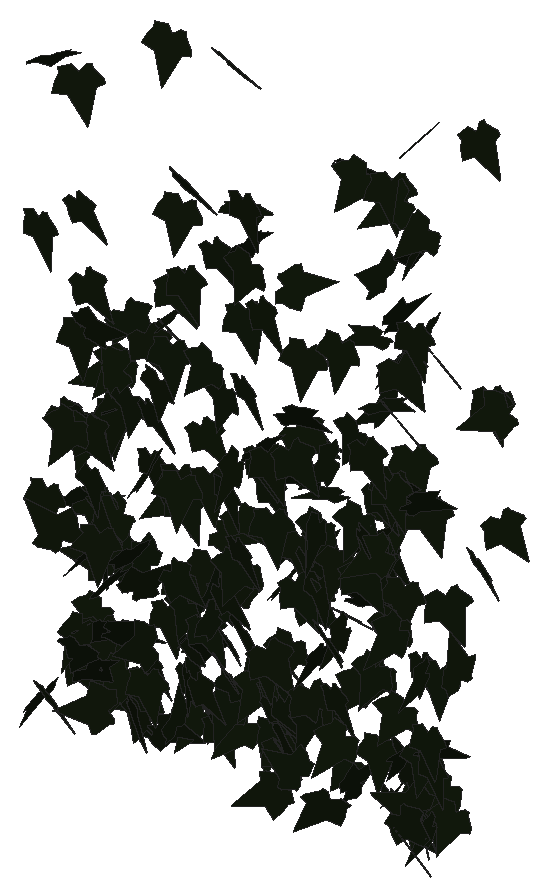
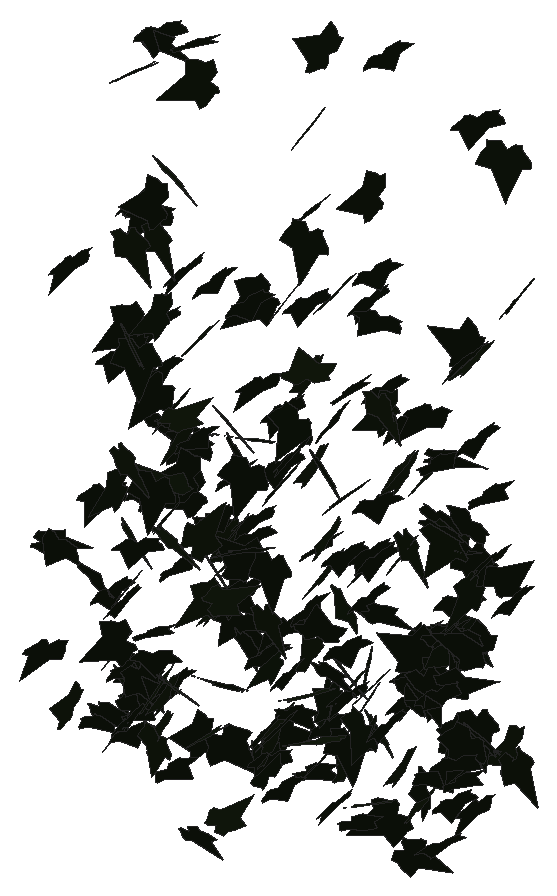
# SketchUp Ruby script. Lengths in inches.
U = 1.inch
M = Sketchup.active_model
def pt(a) = Geom::Point3d.new(a.map { |v| v * U })
def face(e, loops, mat)
  f = e.add_face(loops[0].map { |a| pt(a) })
  loops[1..].each { |l| e.add_face(l.map { |a| pt(a) }).erase! }
  f.material = f.back_material = mat if mat
  f
end
# faces: each face lists its corners as indices into pts; further lists are holes
def faces(e, pts, list, mat = nil) = list.each { |f| face(e, (f[0].is_a?(Array) ? f : [f]).map { |l| l.map { |i| pts[i] } }, mat) }
# xy, xz, yz: faces in a plane at the given z, y or x. An outline is a flat list of corners, or four numbers for a rectangle; further outlines are holes
def ring(l) = l.size == 4 ? [[l[0], l[1]], [l[2], l[1]], [l[2], l[3]], [l[0], l[3]]] : l.each_slice(2).to_a
def flat(e, list, mat, &to3) = list.each { |f| face(e, (f[0].is_a?(Array) ? f : [f]).map { |l| ring(l).map { |u, v| to3.(u, v) } }, mat) }
def xy(e, z, list, mat = nil) = flat(e, list, mat) { |x, y| [x, y, z] }
def xz(e, y, list, mat = nil) = flat(e, list, mat) { |x, z| [x, y, z] }
def yz(e, x, list, mat = nil) = flat(e, list, mat) { |y, z| [x, y, z] }
def lines(e, pts, list) = list.each { |a, b| e.add_line(pt(pts[a]), pt(pts[b])) }
# prism: a flat outline (further loops are holes) pulled along v
def prism(e, loops, v, mat = nil)
  f = face(e, loops, mat); d = Geom::Vector3d.new(v.map { |x| x * U })
  f.pushpull(f.normal.samedirection?(d) ? d.length : -d.length)
end
def box(e, o, s, mat = nil) = prism(e, [[o, [o[0] + s[0], o[1], o[2]], [o[0] + s[0], o[1] + s[1], o[2]], [o[0], o[1] + s[1], o[2]]]], [0, 0, s[2]], mat)
def at(x, y, z, deg = 0) = Geom::Transformation.translation(pt([x, y, z])) * Geom::Transformation.rotation(ORIGIN, Z_AXIS, deg.degrees)
def axes(o, x, y, z) = Geom::Transformation.new([*x, 0, *y, 0, *z, 0, *pt(o).to_a, 1])
def part(name) = M.definitions.add(name)
# library, detail: a bought-in or finely detailed component or shape, given as its bounding box
def library(name, o, s) = part(name).tap { |d| box(d.entities, o, s) }
def detail(e, o, s) = box(e.add_group.entities, o, s)
def put(e, d, t, mat = nil) = e.add_instance(d, t).tap { |i| i.material = mat if mat }
def group(e, t, mat = nil) = e.add_group.tap { |g| g.transformation = t; g.material = mat if mat }.entities
root = M.entities
M.materials.add("efeu1").color = [18, 25, 13]
c1 = part("ivyleaf_9")
p = [[1.54,2.16,1.25],[1.36,2.04,1.19],[-0.21,0.99,0.68],[-0.71,1.11,0.82],[-0.85,0.86,0.67],[-0.8,0.17,0.21],
  [-0.9,-0.01,0.1],[-0.67,-0.16,-0.02],[-0.08,-0.08,-0.05],[-0.03,-0.6,-0.4],[0.65,-0.88,-0.66],[0.83,-0.6,-0.49],
  [1.29,-0.42,-0.43],[1.8125,-0.07,-0.26],[1.21,0.44,0.15]]
faces(c1.entities,p,[[0,1,2,3,4,5,6,7,8,9,10,11,12,13,14]],"efeu1")
put(root,c1,axes([586.22,116.61,357.54],[0.71819,-0.99518,-0.77753],[-0.16369,0.81357,-1.1925],[1.25226,0.6771,0.29005]))
put(root,c1,axes([586.3,123.58,334],[-0.07345,-1.46368,-0.26729],[0.34823,0.24327,-1.42785],[1.44656,-0.13288,0.33015]))
put(root,c1,axes([586.64,118.75,355.34],[1.33189,-0.02046,-0.50214],[-0.4908,0.25288,-1.31212],[0.10806,1.40076,0.22954]))
put(root,c1,axes([587.66,113.28,392.88],[0.45263,1.4208,-0.19565],[-0.46923,-0.04716,-1.42808],[-1.35527,0.49085,0.4291]))
put(root,c1,axes([586.53,118.27,376.59],[0.90416,-1.0969,-0.2869],[0.04377,0.40045,-1.3931],[1.13296,0.85992,0.28278]))
put(root,c1,axes([587.42,120.06,337.79],[-0.70992,-1.06443,0.44559],[-0.10133,-0.46364,-1.26898],[1.14948,-0.69826,0.16333]))
put(root,c1,axes([587.125,113.47,351.75],[0.0436,-1.41863,0.05695],[0.00445,-0.05684,-1.4193],[1.41977,0.04374,0.0027]))
put(root,c1,axes([588.15,117.21,357.48],[0.83336,0.45387,-1.07421],[-0.90735,-0.57701,-0.94772],[-0.73255,1.23104,-0.04816]))
put(root,c1,axes([587.53,117.22,334.38],[0.41458,-0.9867,-0.84246],[-0.20487,0.82354,-1.06536],[1.28115,0.45099,0.10225]))
put(root,c1,axes([587.21,117.31,348.66],[0.5196,-0.16158,1.32532],[1.32539,0.23386,-0.49112],[-0.16095,1.40419,0.2343]))
put(root,c1,axes([589.23,110.3125,334.82],[-0.63267,1.1754,-0.62675],[0.22482,-0.58968,-1.33281],[-1.31295,-0.66735,0.07379]))
put(root,c1,axes([588.08,111.31,378.49],[0.49863,-1.42704,0.04607],[-0.00245,-0.04966,-1.51153],[1.42778,0.49828,-0.01868]))
put(root,c1,axes([588.76,117.14,356.88],[-1.03775,-0.88039,-0.44682],[0.38444,0.23674,-1.35934],[0.90936,-1.10477,0.06478]))
put(root,c1,axes([590.22,117.6,344.51],[-0.65379,0.04671,1.2732],[-1.26249,-0.21614,-0.64036],[0.17128,-1.41484,0.13986]))
put(root,c1,axes([588.86,117.71,349.93],[-0.82625,-0.6682,-0.95212],[0.72316,0.61967,-1.06243],[0.91108,-1.09783,-0.02017]))
put(root,c1,axes([588.67,117.31,352.26],[0.41477,-1.29731,0.38748],[0.11544,-0.36989,-1.362],[1.34901,0.43052,-0.00258]))
put(root,c1,axes([589.17,118.33,334.66],[-0.23341,-1.27695,-0.30092],[0.05641,0.2956,-1.2981],[1.31071,-0.24012,0.00228]))
put(root,c1,axes([589.55,114.96,339.24],[-1.19802,-0.32954,-0.68957],[0.73792,-0.16502,-1.20316],[0.19894,-1.37241,0.31025]))
put(root,c1,axes([589.22,115.3125,366.79],[0.03639,-1.47553,-0.11222],[-0.03578,0.11134,-1.47561],[1.47935,0.03899,-0.03293]))
put(root,c1,axes([589.38,117.78,337.9],[-0.33749,-1.1931,-0.69454],[0.22667,0.6574,-1.23944],[1.3618,-0.4051,0.03418]))
put(root,c1,axes([589.84,115.43,338.71],[0.78837,1.16892,0.14934],[0.07963,0.12643,-1.40993],[-1.17573,0.79237,0.00465]))
put(root,c1,axes([589.78,119.55,344.96],[-0.10207,-1.26752,-0.5716],[0.04327,0.56997,-1.27162],[1.38977,-0.11084,-0.00239]))
put(root,c1,axes([590.11,117.13,358.24],[1.00117,1.09817,0.29768],[-0.05991,0.44685,-1.44695],[-1.13622,0.94408,0.3386]))
put(root,c1,axes([590.17,118.1,349.35],[-0.40572,-1.16314,0.63076],[-0.07215,-0.63932,-1.22533],[1.32119,-0.3921,0.12678]))
put(root,c1,axes([591.28,110.08,350.23],[0.18792,0.30059,1.46884],[-1.48233,0.25923,0.1366],[-0.22482,-1.45795,0.32713]))
put(root,c1,axes([591.62,121.27,330.4375],[-0.2193,-0.15658,-1.36819],[-0.82869,-1.09151,0.25774],[-1.09988,0.8536,0.07861]))
put(root,c1,axes([591.31,117.95,349],[-1.16937,-0.64385,0.53498],[-0.46293,-0.26836,-1.33486],[0.69745,-1.25762,0.01095]))
put(root,c1,axes([590.69,112.47,359.73],[-0.61427,-1.2618,0.47841],[-0.10896,-0.47755,-1.39944],[1.34505,-0.61494,0.10512]))
put(root,c1,axes([589.83,109.71,335.49],[1.16984,-0.88217,0.28166],[0.23188,-0.16031,-1.46513],[0.89655,1.19254,0.01141]))
put(root,c1,axes([591.32,112.62,338.86],[0.76274,0.60119,-1.10895],[-0.96426,-0.55762,-0.96552],[-0.81326,1.22499,0.10473]))
put(root,c1,axes([590.06,127.95,338.22],[-0.05013,-1.39465,-0.24492],[0.77061,0.17873,-1.17548],[1.18794,-0.1748,0.7522]))
put(root,c1,axes([591.68,118.86,345.28],[-0.16332,1.30316,-0.58109],[-0.03806,-0.58866,-1.30942],[-1.42634,-0.13351,0.10148]))
put(root,c1,axes([591.88,113.99,347.84],[-0.72942,1.02361,-0.70913],[0.04516,-0.79955,-1.20058],[-1.24443,-0.629,0.37209]))
put(root,c1,axes([590.64,116.51,344.31],[-0.09897,0.18185,1.45176],[0.32329,-1.4164,0.19946],[1.42694,0.33352,0.05551]))
put(root,c1,axes([590.97,117.73,358.95],[-0.86623,-0.79984,-0.90298],[0.92176,0.2782,-1.13067],[0.77812,-1.21997,0.33418]))
put(root,c1,axes([590.46,114.52,358.34],[-0.13441,-0.56577,-1.35578],[1.18838,0.75854,-0.43436],[0.8637,-1.13174,0.38665]))
put(root,c1,axes([592.55,120,343.84],[-0.46042,0.32471,1.30651],[-1.07342,0.74482,-0.56339],[-0.81251,-1.16799,0.00394]))
put(root,c1,axes([591.2,113.52,373],[0.66268,-1.15667,-0.60639],[-0.03577,0.66366,-1.305],[1.30549,0.60532,0.27205]))
put(root,c1,axes([591.79,117.18,359.67],[-1.16008,-0.43014,-0.81683],[0.77741,0.25228,-1.23694],[0.49786,-1.39619,0.02814]))
put(root,c1,axes([592.93,115.95,363.93],[-1.22716,-0.12721,0.85092],[-0.80276,-0.36399,-1.21213],[0.30955,-1.44827,0.2299]))
put(root,c1,axes([592.32,117.07,364.11],[-0.79306,-1.07983,0.55135],[-0.20758,-0.52817,-1.33301],[1.19455,-0.80868,0.1344]))
put(root,c1,axes([592.28,112.46,337.17],[0.79684,1.17437,0.25341],[0.11681,0.2269,-1.41887],[-1.1957,0.80479,0.03026]))
put(root,c1,axes([592.15,111.47,393.59],[-0.31415,-1.32015,-0.67244],[0.17383,0.6498,-1.35691],[1.47131,-0.35864,0.01674]))
put(root,c1,axes([592.7,116.78,335.25],[-0.86334,-1.22428,0.02958],[-0.01057,-0.02874,-1.49805],[1.22459,-0.86337,0.00792]))
put(root,c1,axes([592.96,113.13,349.7],[-0.45901,-1.28293,-0.40304],[0.1232,0.38397,-1.36251],[1.33909,-0.47508,-0.0128]))
put(root,c1,axes([592.61,116.99,368.77],[0.22659,-0.81784,-1.18014],[0.18579,1.2014,-0.7969],[1.42375,-0.02662,0.29181]))
put(root,c1,axes([593.49,112.73,345.13],[0.54595,0.90484,1.05669],[0.21228,1.06766,-1.02392],[-1.37486,0.52415,0.26151]))
put(root,c1,axes([594.45,112.05,334.28],[-0.83948,-0.18439,1.19989],[-1.13496,-0.39852,-0.85529],[0.43083,-1.40913,0.08488]))
put(root,c1,axes([593.3,128.61,343.36],[1.22881,-0.55122,-0.41885],[0.3017,1.1944,-0.68674],[0.6231,0.50872,1.15853]))
put(root,c1,axes([593.81,117.28,331.58],[-0.05729,-1.07996,0.85608],[0.25628,-0.85023,-1.05542],[1.35407,0.11523,0.23597]))
put(root,c1,axes([593.93,116.16,361.6],[0.02406,-1.2772,0.64928],[0.19948,-0.64006,-1.26646],[1.41881,0.11165,0.16705]))
put(root,c1,axes([595.4,120.93,351.04],[-1.22157,-0.39612,0.48577],[-0.46186,-0.15052,-1.28419],[0.42375,-1.30597,0.00067]))
put(root,c1,axes([594.05,118.37,336.25],[0.87876,-1.00952,-0.04734],[-0.02769,0.03866,-1.33841],[1.01025,0.87919,0.00449]))
put(root,c1,axes([595.72,116.36,355.59],[-0.95245,1.0759,-0.2968],[0.20577,-0.21422,-1.43686],[-1.09695,-0.97436,-0.01183]))
put(root,c1,axes([594.18,115.65,332.76],[-0.01391,0.03691,-1.4553],[1.45574,0.0082,-0.01371],[0.00785,-1.45534,-0.03698]))
put(root,c1,axes([594.02,110.16,370.88],[0.51863,-0.22234,1.37144],[1.23485,-0.59711,-0.56379],[0.63673,1.33913,-0.02368]))
put(root,c1,axes([594.59,117.94,355.4],[0.57722,-1.29926,0.06332],[0.02392,-0.05866,-1.42171],[1.30059,0.57772,-0.00195]))
put(root,c1,axes([594.84,119.82,340.4],[0.22889,-1.3565,-0.16098],[-0.0017,0.16294,-1.37544],[1.36601,0.22749,0.02526]))
put(root,c1,axes([594.8125,117.05,367.39],[0.29106,-1.201,-0.72711],[0.18321,0.76872,-1.19638],[1.39196,0.14995,0.30951]))
put(root,c1,axes([596.44,118.73,369.22],[-0.60027,1.30334,0.11699],[-0.30422,-0.01381,-1.40712],[-1.27273,-0.61141,0.28116]))
put(root,c1,axes([595.07,118.26,362.64],[0.16605,-1.25244,0.68003],[0.20928,-0.65578,-1.25887],[1.40969,0.24489,0.10679]))
put(root,c1,axes([595.11,115.16,344.48],[0.11476,-0.21163,1.43679],[1.36908,0.49664,-0.0362],[-0.48455,1.3531,0.238]))
put(root,c1,axes([595.24,112.08,341.9],[1.18145,0.239,0.91451],[0.87298,0.28542,-1.20239],[-0.36244,1.46653,0.08497]))
put(root,c1,axes([595.67,117.72,330.75],[0.06905,0.21885,-1.43136],[0.55156,1.32098,0.22858],[1.33883,-0.55549,-0.02035]))
put(root,c1,axes([596.18,120.57,351.99],[0.06787,-1.36175,-0.14946],[-0.0087,0.14921,-1.36344],[1.3699,0.06842,-0.00126]))
put(root,c1,axes([595.98,115.74,361.63],[1.05883,-1.02786,-0.12884],[-0.05951,0.12358,-1.47492],[1.03419,1.05946,0.04704]))
put(root,c1,axes([595.92,118.14,368.18],[1.27409,-0.60733,0.25545],[0.26186,-0.04354,-1.40959],[0.60459,1.29872,0.0722]))
put(root,c1,axes([597.3125,119.67,339.2],[0.13338,1.21568,0.7693],[-0.04756,0.7759,-1.21787],[-1.43786,0.0871,0.11164]))
put(root,c1,axes([595.94,127.86,346.26],[0.6012,-1.23103,-0.37042],[0.63406,0.63968,-1.09676],[1.11831,0.29912,0.82098]))
put(root,c1,axes([597.37,120.99,331.01],[-0.90845,-0.9713,0.2073],[-0.0564,-0.23003,-1.32498],[0.99157,-0.90296,0.11455]))
put(root,c1,axes([596.89,118.61,354.49],[0.10619,-1.39244,-0.29469],[-0.03417,0.29293,-1.39643],[1.42287,0.11095,-0.01154]))
put(root,c1,axes([596.58,127.91,375.36],[-0.29007,-1.43899,0.38433],[1.17655,-0.46147,-0.83983],[0.9133,0.13746,1.20396]))
put(root,c1,axes([598.15,120.41,338.24],[0.37869,1.19675,-0.49344],[-0.21519,-0.44877,-1.25355],[-1.27647,0.43069,0.06494]))
put(root,c1,axes([597.46,119.0625,342.15],[-0.16987,-1.19487,0.69858],[0.13361,-0.71469,-1.18994],[1.37763,-0.07802,0.20155]))
put(root,c1,axes([597.24,119.77,337.9],[0.43448,-1.13903,0.66149],[0.22676,-0.62146,-1.21905],[1.29751,0.49002,-0.00845]))
put(root,c1,axes([597.82,117.86,380.34],[-0.4341,-1.39095,-0.09361],[0.02466,0.09036,-1.45711],[1.39387,-0.43479,-0.00337]))
put(root,c1,axes([598.38,112.65,338.41],[0.08376,-1.39141,-0.30198],[0.01948,0.30359,-1.39344],[1.42367,0.0777,0.03683]))
put(root,c1,axes([598.63,115.55,368.27],[-0.09613,-1.44563,-0.17645],[0.02497,0.17517,-1.44876],[1.45615,-0.09844,0.0132]))
put(root,c1,axes([598.98,120.16,346.22],[-0.43427,-1.31166,-0.15494],[0.03289,0.15231,-1.38159],[1.32037,-0.4352,-0.01654]))
put(root,c1,axes([599.49,111.63,342.22],[-0.45485,-0.48635,1.32151],[-0.64146,-1.16472,-0.64944],[1.25358,-0.77246,0.14718]))
put(root,c1,axes([598.8,116.91,353.75],[0.20587,-1.34072,-0.43835],[0.0723,0.45244,-1.34986],[1.40871,0.17271,0.13334]))
put(root,c1,axes([599.42,114.5,398.35],[-0.37937,-1.46477,0.04473],[-0.00666,-0.04448,-1.51309],[1.46544,-0.3794,0.0047]))
put(root,c1,axes([599.3,119.66,354.57],[-0.11988,-1.35425,-0.37068],[0.09334,0.36352,-1.35827],[1.40095,-0.1401,0.05878]))
put(root,c1,axes([599,115.55,374.62],[-0.24017,-0.98003,-1.02974],[0.80127,0.7693,-0.91904],[1.17421,-0.72541,0.41653]))
put(root,c1,axes([599.38,118.9,341.28],[0.33076,-1.22251,-0.58126],[0.04295,0.60754,-1.25334],[1.35298,0.27958,0.18189]))
put(root,c1,axes([599.45,118.58,359.67],[0.65155,-1.18582,-0.46502],[0.13358,0.58306,-1.29966],[1.26671,0.54846,0.37624]))
put(root,c1,axes([601.12,113.13,334.8],[-1.11212,0.5975,-0.80749],[-0.73591,0.33534,1.26168],[0.68372,1.33281,0.04455]))
put(root,c1,axes([599.89,120.03,331.43],[0.4062,-1.22151,-0.33495],[0.01537,0.35648,-1.28139],[1.2665,0.38745,0.12298]))
put(root,c1,axes([601.19,120.0625,343.4375],[-1.35913,-0.13324,-0.0068],[0.0076,-0.00781,-1.36562],[0.13319,-1.35913,0.00851]))
put(root,c1,axes([600.36,114.53,356.7],[-0.45459,-1.33089,-0.26563],[0.12181,0.23899,-1.40589],[1.35166,-0.46914,0.03736]))
put(root,c1,axes([599.8,118.5,334.08],[0.36086,-0.99137,0.89218],[0.51927,-0.7469,-1.03996],[1.22848,0.60692,0.17751]))
put(root,c1,axes([601.45,117.88,342.93],[-1.19388,0.63723,0.09578],[-0.09041,0.03402,-1.35324],[-0.63801,-1.19723,0.01253]))
put(root,c1,axes([600.3,115.4,338.71],[0.87639,-1.01627,-0.57294],[-0.36824,0.439,-1.34194],[1.10701,0.95058,0.0072]))
put(root,c1,axes([600.3,115.1875,375.79],[0.26162,-1.37055,-0.38286],[0.00209,0.38965,-1.39341],[1.42302,0.2514,0.07243]))
put(root,c1,axes([599.95,128.96,368.73],[1.31934,-0.46118,-0.45248],[0.40093,1.39118,-0.24892],[0.50664,0.10007,1.37528]))
put(root,c1,axes([599.98,114.71,385.09],[1.2909,-0.59225,0.48479],[0.44592,-0.19058,-1.42023],[0.62204,1.3657,0.01204]))
put(root,c1,axes([601.08,120.64,335.12],[0.04252,-1.26087,0.50961],[0.11276,-0.50483,-1.25846],[1.35528,0.08156,0.08872]))
put(root,c1,axes([601.56,116.9,367.27],[-0.55287,-1.07256,0.79441],[-0.08161,-0.8311,-1.17888],[1.33222,-0.49602,0.25747]))
put(root,c1,axes([600.73,119.81,340.05],[0.50438,-0.88301,0.95682],[0.53779,-0.79319,-1.0155],[1.18574,0.73536,0.05357]))
put(root,c1,axes([601.15,117.94,377.52],[0.78896,-1.17861,-0.33272],[0.00421,0.39839,-1.40126],[1.22466,0.75792,0.21916]))
put(root,c1,axes([602.96,115.02,346.54],[-0.96171,0.65482,-0.93734],[-0.76198,0.54618,1.16334],[0.85252,1.22686,-0.01761]))
put(root,c1,axes([601.57,118.93,354.7],[0.61757,-1.22369,0.35614],[0.13976,-0.32834,-1.37052],[1.26678,0.63279,-0.02242]))
put(root,c1,axes([602.08,111.41,350.14],[0.80262,-0.82109,-0.89977],[-0.29012,0.91767,-1.09621],[1.18304,0.78209,0.34161]))
put(root,c1,axes([602.37,117.84,364.51],[0.03736,-1.28682,0.66912],[-0.01362,-0.66962,-1.28703],[1.45032,0.02686,-0.02932]))
put(root,c1,axes([603.13,118.26,345.05],[-1.27065,-0.26749,0.60784],[0.60628,0.06827,1.29744],[-0.27101,1.4069,0.05261]))
put(root,c1,axes([603.3,119.35,332.86],[-1.00201,-0.86953,0.39492],[-0.20524,-0.36297,-1.31993],[0.9327,-1.01402,0.13382]))
put(root,c1,axes([602.23,113.06,339.75],[0.21383,-0.0716,-1.40799],[1.29322,-0.55709,0.22473],[-0.56136,-1.31065,-0.01861]))
put(root,c1,axes([602.4375,118.05,337.77],[-0.30053,-0.45039,1.24694],[0.51662,-1.21729,-0.31516],[1.22098,0.4042,0.44027]))
put(root,c1,axes([602.76,113.92,338.89],[0.87781,-0.99672,-0.47626],[-0.17944,0.47159,-1.31766],[1.08999,0.88033,0.16663]))
put(root,c1,axes([602.67,127.11,357],[0.72051,-1.05566,-0.70857],[0.60838,1.00141,-0.87332],[1.11641,0.13559,0.93321]))
put(root,c1,axes([603.58,116.89,335.91],[-0.40942,-1.2876,0.23439],[-0.05429,-0.22867,-1.35101],[1.30763,-0.41264,0.01729]))
put(root,c1,axes([603.6,119.375,347.67],[-0.20179,-1.3009,0.4104],[-0.10853,-0.39824,-1.31572],[1.35978,-0.22484,-0.04411]))
put(root,c1,axes([604.92,116.01,359.33],[-1.31938,0.17367,-0.70505],[0.70025,-0.08253,-1.33074],[-0.1921,-1.49367,-0.00845]))
put(root,c1,axes([604.11,127.68,343.85],[1.37251,-0.00247,-0.11335],[0.00772,1.3757,0.06349],[0.11311,-0.06391,1.37105]))
put(root,c1,axes([604.03,118.07,342.55],[0.23289,-0.9554,1.01097],[0.49782,-0.8999,-0.96512],[1.29886,0.51622,0.18863]))
put(root,c1,axes([604.6,121.4,331.76],[-0.29394,-1.31968,0.07818],[0.00031,-0.08016,-1.3519],[1.32199,-0.29341,0.0177]))
put(root,c1,axes([605.4,131.82,331.91],[-1.29165,-0.31756,-0.00579],[0.00506,0.00366,-1.33011],[0.31757,-1.29166,-0.00234]))
put(root,c1,axes([605.29,119.19,337.62],[-1.06053,-0.84527,-0.02285],[0.07603,-0.05881,-1.35296],[0.84215,-1.05914,0.09337]))
put(root,c1,axes([605.8,128.24,351.45],[-1.39825,-0.11002,0.07848],[0.07354,-1.30382,-0.51769],[0.11339,-0.51118,1.30353]))
put(root,c1,axes([605.72,116.27,380.27],[0.30483,1.43413,0.09242],[-0.01928,0.09855,-1.46564],[-1.43697,0.3029,0.03928]))
put(root,c1,axes([605.69,127.93,330.96],[-1.23613,-0.40955,0.37513],[0.28935,-1.2562,-0.418],[0.47406,-0.30119,1.2333]))
put(root,c1,axes([604.41,115.64,397.17],[0.73585,-0.88931,0.97074],[0.89207,-0.48104,-1.11691],[0.9682,1.11911,0.29131]))
put(root,c1,axes([606.59,120.85,346.91],[-0.72058,1.16773,-0.10601],[-0.02677,-0.14078,-1.36877],[-1.17223,-0.7146,0.09642]))
put(root,c1,axes([605.32,113.64,348.73],[1.00136,-0.86999,-0.55666],[-0.26974,0.52813,-1.31064],[0.99699,1.01669,0.20449]))
put(root,c1,axes([605.3,120.29,336.86],[0.69871,-1.09307,-0.48421],[-0.076,0.51909,-1.28149],[1.1931,0.67319,0.20193]))
put(root,c1,axes([606.46,120.1,351.33],[0.91444,0.51736,-0.92018],[-0.81404,-0.4295,-1.05045],[-0.6721,1.22412,0.02033]))
put(root,c1,axes([605.99,115.07,350.58],[-0.40596,-1.27659,0.53916],[0.06376,-0.57843,-1.32156],[1.38431,-0.34773,0.21898]))
put(root,c1,axes([605.63,116.01,367.18],[0.89593,-1.1274,0.1164],[0.04807,-0.11044,-1.43971],[1.13237,0.89668,-0.03097]))
put(root,c1,axes([605.99,116.07,374.01],[-0.03955,-1.37857,-0.49737],[0.09439,0.49412,-1.37707],[1.4625,-0.06918,0.07542]))
put(root,c1,axes([606.04,118.36,340.6],[0.22459,-1.36089,-0.08072],[0.00281,0.08227,-1.3792],[1.36328,0.22403,0.01614]))
put(root,c1,axes([606.47,117.23,360.27],[0.55881,-1.30448,-0.29792],[-0.03777,0.30735,-1.41662],[1.33753,0.55368,0.08447]))
put(root,c1,axes([606.45,118.74,336.3],[0.94682,-0.90171,-0.3328],[-0.079,0.39257,-1.28839],[0.95791,0.92364,0.22269]))
put(root,c1,axes([608,132.21,358.8125],[-1.19401,0.7644,0.03517],[-0.19015,-0.23325,-1.38588],[-0.74121,-1.17154,0.29887]))
put(root,c1,axes([607.6,115.43,362],[0.55196,1.22692,0.44872],[0.06893,0.45909,-1.34008],[-1.30458,0.54336,0.11904]))
put(root,c1,axes([607.06,119.94,335.76],[0.54639,-1.32625,-0.23181],[-0.07173,0.22114,-1.43429],[1.34444,0.5508,0.01768]))
put(root,c1,axes([607.11,116.51,374.63],[0.80468,-1.19179,-0.37751],[-0.15899,0.34775,-1.43672],[1.24,0.81799,0.06077]))
put(root,c1,axes([607.11,117.62,357.75],[0.68624,-1.23226,-0.32982],[-0.07836,0.33309,-1.40751],[1.27323,0.68465,0.09114]))
put(root,c1,axes([607.14,118.55,341.5],[1.27545,-0.59538,-0.15496],[-0.1313,0.08505,-1.40741],[0.60104,1.28201,0.0214]))
put(root,c1,axes([608.4375,131.8125,345.12],[-1.3583,0.15742,-0.14989],[0.10863,-0.32998,-1.33099],[-0.18827,-1.3261,0.3134]))
put(root,c1,axes([607.6,134,348.52],[-0.68893,-1.08738,-0.52082],[0.42424,0.34285,-1.277],[1.12856,-0.79267,0.16211]))
put(root,c1,axes([607.43,118.93,332.53],[-0.01751,-1.13637,-0.71638],[0.14688,0.71053,-1.13067],[1.33528,-0.09305,0.11498]))
put(root,c1,axes([608.26,127.81,355.77],[-1.31757,-0.23029,0.5296],[0.30879,-1.39576,0.1613],[0.48802,0.26141,1.32778]))
put(root,c1,axes([607.38,119.34,333.15],[0.34036,-0.97262,0.88434],[0.31195,-0.82765,-1.03033],[1.277,0.46142,0.01599]))
put(root,c1,axes([608.02,119.5,341.96],[-0.46264,-1.28753,0.21412],[-0.03851,-0.21361,-1.36766],[1.30464,-0.46287,0.03556]))
put(root,c1,axes([607.54,132.04,344.25],[0.94251,-0.99178,-0.08584],[-0.0588,0.06253,-1.3682],[0.99375,0.94434,0.00045]))
put(root,c1,axes([607.85,132.33,345.33],[0.88933,-0.9189,-0.50596],[-0.32044,0.39363,-1.27814],[0.99885,0.94443,0.04044]))
put(root,c1,axes([607.43,119.37,331.14],[0.18363,-0.67474,1.26436],[0.80171,-1.00821,-0.65448],[1.18791,0.78474,0.24626]))
put(root,c1,axes([608.13,113.91,380.08],[-0.33308,-1.27835,0.70772],[0.09337,-0.74302,-1.29815],[1.45819,-0.24442,0.24478]))
put(root,c1,axes([608.72,132.28,363.19],[0.32695,1.39426,-0.04868],[0.01772,-0.05415,-1.43178],[-1.395,0.32609,-0.0296]))
put(root,c1,axes([609.46,129.08,367.24],[-1.32103,-0.45592,0.38813],[0.2487,-1.27305,-0.64893],[0.54466,-0.5245,1.23769]))
put(root,c1,axes([608.57,115.6875,343.11],[0.21981,-1.15176,-0.93886],[0.17381,0.96249,-1.14006],[1.47573,0.05819,0.27411]))
put(root,c1,axes([609.34,119.47,358.61],[0.69871,1.22453,-0.12666],[-0.05645,-0.11362,-1.40983],[-1.22977,0.70095,-0.00725]))
put(root,c1,axes([609.39,129.7,335.48],[-0.6417,-1.15165,0.34518],[-0.19269,-0.28769,-1.31808],[1.18673,-0.66945,-0.02737]))
put(root,c1,axes([608.94,112.03,387.22],[0.61798,-1.38471,0.05444],[0.01782,-0.05166,-1.51634],[1.38566,0.61822,-0.00478]))
put(root,c1,axes([608.97,120.1,350.04],[-0.06414,-0.42074,1.32367],[1.33957,0.3314,0.17024],[-0.367,1.28312,0.39006]))
put(root,c1,axes([609.36,119.1,352.41],[-0.15754,-1.35733,-0.37921],[0.1783,0.35931,-1.36017],[1.39798,-0.19879,0.13075]))
put(root,c1,axes([609.43,114.74,362.33],[0.17104,-1.33042,-0.62015],[-0.07583,0.61551,-1.34136],[1.46589,0.18707,0.00297]))
put(root,c1,axes([609.22,110.92,355.46],[0.92178,-1.13065,0.0773],[0.02965,-0.07555,-1.45857],[1.1329,0.92193,-0.02472]))
put(root,c1,axes([610.5625,114.68,331.42],[-0.11332,-0.52776,-1.3271],[-0.03812,-1.32968,0.53204],[-1.42768,0.07739,0.09113]))
put(root,c1,axes([610.81,134.09,366.04],[-1.01581,0.9717,-0.31128],[0.13407,-0.30832,-1.39998],[-1.0115,-1.01672,0.12704]))
put(root,c1,axes([610.82,131.83,374.5625],[0.28413,1.42331,-0.22],[-0.22617,-0.17736,-1.43956],[-1.42234,0.31253,0.18496]))
put(root,c1,axes([609.82,119.4,351.3],[0.93598,-0.96297,-0.44928],[-0.12054,0.49863,-1.31987],[1.05576,0.91065,0.24761]))
put(root,c1,axes([610.11,114.4,356.8],[-0.04781,-1.41611,-0.37192],[-0.01623,0.37261,-1.41665],[1.46405,-0.04211,-0.02785]))
put(root,c1,axes([611.36,132.41,385.05],[-0.60551,1.36107,-0.18474],[-0.12115,-0.25403,-1.47447],[-1.36819,-0.57986,0.21233]))
put(root,c1,axes([609.58,129.21,360.89],[0.54531,-1.28181,0.32044],[1.25488,0.39396,-0.55961],[0.41352,0.49482,1.27564]))
put(root,c1,axes([610.21,118.95,347.47],[0.47658,-0.87766,-1.00415],[-0.06705,1.04922,-0.94888],[1.33195,0.36685,0.31152]))
put(root,c1,axes([610.26,134.88,363.61],[1.33768,-0.48117,-0.14529],[-0.12585,0.07928,-1.42123],[0.48661,1.34321,0.03184]))
put(root,c1,axes([611.2,132.78,376],[-1.18357,0.33322,-0.80903],[0.77116,-0.24571,-1.22936],[-0.41338,-1.41244,0.02299]))
put(root,c1,axes([611.8,116.78,372.04],[-0.33067,-1.41671,-0.06953],[0.01603,0.06765,-1.45479],[1.41832,-0.33106,0.00023]))
put(root,c1,axes([611.625,130.9375,356.07],[-0.36687,-1.19212,-0.66899],[0.3719,0.5795,-1.23659],[1.31544,-0.49631,0.16303]))
put(root,c1,axes([612.05,114.43,363.66],[0.35858,-1.16255,-0.85228],[0.08591,0.89393,-1.18322],[1.43894,0.23634,0.28303]))
put(root,c1,axes([613.48,118.04,361.75],[-1.36142,0.48171,-0.02484],[0.01519,-0.03153,-1.44392],[-0.48211,-1.36128,0.02465]))
put(root,c1,axes([612.28,120.26,346.26],[1.38598,0.09916,-0.0159],[-0.04334,0.39206,-1.33246],[-0.09059,1.32947,0.39413]))
put(root,c1,axes([612.36,114.79,351.18],[0.3456,-1.27743,-0.64256],[0.03585,0.6686,-1.3099],[1.42948,0.29207,0.1882]))
put(root,c1,axes([612.9,117.36,355.82],[-0.3527,-1.27966,0.46207],[-0.04223,-0.46682,-1.32505],[1.35988,-0.34639,0.0787]))
put(root,c1,axes([612.84,117.11,350.48],[0.38486,-1.33659,0.25682],[0.03818,-0.25618,-1.39048],[1.3605,0.38528,-0.03363]))
put(root,c1,axes([613.69,116.33,344.73],[-0.56787,0.55902,-1.13845],[0.55229,-1.01388,-0.77335],[-1.14173,-0.76849,0.19215]))
put(root,c1,axes([613.43,118.92,352.63],[-0.384,-1.37574,0.05416],[0.00274,-0.057,-1.42822],[1.37681,-0.38359,0.01795]))
put(root,c1,axes([614.37,116.41,330.78],[0.13709,0.50986,-1.36194],[-0.48522,-1.27355,-0.52561],[-1.37091,0.50175,0.04985]))
put(root,c1,axes([613.82,114.78,339.64],[-1.25778,-0.15183,-0.71672],[0.70531,0.13426,-1.2662],[0.19818,-1.44141,-0.04244]))
put(root,c1,axes([613.67,120.29,332.5],[-0.62101,-1.01482,0.65794],[0.18688,-0.81124,-1.07488],[1.19491,-0.40054,0.51004]))
put(root,c1,axes([613,137.76,343.4],[0.80653,-0.97014,0.58857],[0.35209,-0.4725,-1.2613],[1.07872,0.87958,-0.02838]))
put(root,c1,axes([613.5625,136.94,384.27],[0.38793,-1.20275,-0.8016],[-0.12859,0.79796,-1.25952],[1.43967,0.39537,0.1035]))
put(root,c1,axes([613.7,138.56,358.91],[-0.66231,-0.58137,-1.13518],[0.97687,0.59112,-0.87268],[0.81997,-1.17382,0.12276]))
put(root,c1,axes([614.2,115.24,357.13],[-1.12405,0.08151,-0.97216],[0.97023,-0.0615,-1.12698],[-0.10189,-1.48485,-0.00669]))
put(root,c1,axes([613.73,114.87,341.5],[-0.15057,-0.99929,-1.02047],[0.41706,0.95064,-0.99245],[1.36602,-0.40038,0.19052]))
put(root,c1,axes([615.58,138.24,358.08],[-1.0878,-0.38406,0.87005],[-0.77745,-0.40224,-1.14959],[0.54776,-1.3336,0.09618]))
put(root,c1,axes([615.89,110.51,336.37],[-0.41658,0.42238,1.24961],[-1.18182,0.46251,-0.55031],[-0.58586,-1.23334,0.22158]))
put(root,c1,axes([614.21,111.38,369.37],[1.30755,0.58379,0.43393],[0.38378,0.20459,-1.43166],[-0.61792,1.3624,0.02905]))
put(root,c1,axes([614.77,117.62,373.27],[-0.16125,-1.42825,0.19482],[-0.00124,-0.1959,-1.43718],[1.44148,-0.15994,0.02055]))
put(root,c1,axes([615.54,116.9375,347.08],[-1.27117,0.33638,-0.48656],[0.48007,-0.08711,-1.31443],[-0.34559,-1.35832,-0.0362]))
put(root,c1,axes([615,118.27,331.32],[0.13001,0.21997,1.39178],[0.80208,1.1376,-0.25472],[-1.1585,0.8123,-0.02016]))
put(root,c1,axes([615.51,137.68,348.14],[0.18876,-0.9415,-1.05401],[0.00357,1.06368,-0.9495],[1.41327,0.12306,0.14317]))
put(root,c1,axes([615.57,114.66,347.29],[0.42606,-0.96732,1.05916],[0.61756,-0.87355,-1.04622],[1.29466,0.73502,0.15049]))
put(root,c1,axes([615.93,115.07,342.14],[0.86138,-1.14204,-0.12492],[-0.06369,0.10842,-1.43039],[1.14709,0.86361,0.01438]))
put(root,c1,axes([615.76,116.76,391.03],[1.37033,0.02019,0.57035],[0.54392,0.403,-1.32108],[-0.17281,1.42853,0.36463]))
put(root,c1,axes([616.66,117.73,354.6],[0.38197,0.29617,1.38633],[0.86002,1.09297,-0.47045],[-1.12694,0.93447,0.11087]))
put(root,c1,axes([616.93,117.49,357.9],[-0.46202,-1.30272,0.30419],[-0.07177,-0.29722,-1.38187],[1.33584,-0.46653,0.03097]))
put(root,c1,axes([617.14,116.68,366.27],[-0.28544,-1.11664,0.90899],[0.13273,-0.94314,-1.11691],[1.43371,-0.135,0.28437]))
put(root,c1,axes([618.07,120.39,331.13],[-0.0299,1.1823,0.56334],[-0.08532,0.56053,-1.18094],[-1.30687,-0.06365,0.06421]))
put(root,c1,axes([617.67,119.11,335.96],[-0.09425,-1.39177,0.02875],[0.00465,-0.02913,-1.39495],[1.39206,-0.09413,0.00661]))
put(root,c1,axes([617.85,118.83,351.5],[0.59614,-1.26435,-0.1792],[-0.03552,0.18127,-1.39712],[1.27649,0.59552,0.04482]))
put(root,c1,axes([619.79,116.99,381.64],[-0.86123,0.97795,0.69685],[-0.60375,0.38864,-1.29158],[-1.03802,-1.03744,0.17305]))
put(root,c1,axes([618.3,117.68,360.77],[0.72875,-1.13378,-0.45794],[-0.15582,0.44265,-1.34389],[1.2128,0.73814,0.10251]))
put(root,c1,axes([618.11,115.37,351.73],[1.15224,0.21532,0.78492],[0.70571,0.41349,-1.1494],[-0.4055,1.33146,0.23001]))
put(root,c1,axes([618.32,119.6,331.38],[0.72929,-1.09657,0.29524],[0.16415,-0.24541,-1.31695],[1.1237,0.74754,0.00076]))
put(root,c1,axes([618.63,115.6,357.65],[1.21958,-0.70142,-0.48697],[-0.39864,0.28316,-1.40621],[0.75513,1.28232,0.04415]))
put(root,c1,axes([619.49,114.7,392.26],[-0.9342,-1.09073,0.49098],[0.05915,-0.66435,-1.36332],[1.19468,-0.82002,0.45143]))
put(root,c1,axes([619.31,116.68,344.9],[-0.39705,-1.23988,0.48188],[-0.0847,-0.4783,-1.30046],[1.32753,-0.40135,0.06116]))
put(root,c1,axes([619.68,119.54,339.95],[-0.81363,-1.05901,0.39058],[0.06793,-0.52654,-1.28615],[1.12669,-0.73301,0.35959]))
put(root,c1,axes([620.43,119.58,336.14],[-0.19233,1.0084,-0.84269],[-0.0661,-0.85801,-1.01165],[-1.31249,-0.10455,0.17444]))
put(root,c1,axes([620.84,119.38,334.16],[0.00088,-0.02103,1.42557],[-0.90129,1.10458,0.01685],[-1.10471,-0.9012,-0.01261]))
put(root,c1,axes([619.3,117.96,368.84],[1.275,-0.65604,0.19068],[0.17339,-0.07978,-1.43386],[0.66082,1.28671,0.00832]))
put(root,c1,axes([619.8,117.86,361.93],[1.31883,0.59296,-0.04033],[-0.03818,-0.01344,-1.44599],[-0.5931,1.31938,0.00339]))
put(root,c1,axes([619.625,114.01,355.48],[-0.33644,-0.73611,-1.20925],[0.76234,0.95312,-0.7923],[1.19289,-0.81673,0.16528]))
put(root,c1,axes([621.1,115.15,357.0625],[-1.33003,-0.32152,0.3936],[-0.2927,-0.41686,-1.3296],[0.41548,-1.32293,0.32331]))
put(root,c1,axes([620.49,117.24,362.93],[-0.04596,-1.44786,-0.0496],[-0.0533,0.05128,-1.44755],[1.44773,-0.04407,-0.05487]))
put(root,c1,axes([620.72,116.74,377.94],[0.41509,0.31737,1.37767],[0.80809,1.12489,-0.50261],[-1.16004,0.89716,0.14284]))
put(root,c1,axes([621.71,116.08,374.78],[-0.77636,1.20987,-0.23901],[0.14145,-0.1932,-1.43746],[-1.22511,-0.78901,-0.01451]))
put(root,c1,axes([620.625,120.85,332.3],[0.1435,-1.35729,0.14133],[0.00731,-0.14134,-1.36483],[1.3646,0.14349,-0.00755]))
put(root,c1,axes([622.02,118.58,331.65],[-0.27318,0.00404,1.42058],[-1.37311,-0.3716,-0.26299],[0.36418,-1.39806,0.07401]))
put(root,c1,axes([621.03,118.1,352.37],[-0.29817,-1.34633,-0.23267],[0.0337,0.23083,-1.37885],[1.36587,-0.2996,-0.01677]))
put(root,c1,axes([620.79,120.7,344.33],[0.60543,-1.21547,-0.14231],[-0.04816,0.13498,-1.3578],[1.22282,0.60711,0.01698]))
put(root,c1,axes([621.25,120.09,330.53],[-0.48186,-1.22323,-0.06714],[0.08867,0.03714,-1.31292],[1.22186,-0.48509,0.0688]))
put(root,c1,axes([621.74,116.14,350.26],[-0.55322,-1.27362,0.34792],[-0.0998,-0.33581,-1.38798],[1.31651,-0.56066,0.04098]))
put(root,c1,axes([621.68,120.11,336.4],[-0.3326,-1.3287,0.08853],[-0.01019,-0.08871,-1.36965],[1.33161,-0.33256,0.01163]))
put(root,c1,axes([621.53,121.21,330.66],[0.24923,-1.23586,0.4161],[0.09424,-0.40546,-1.26069],[1.30062,0.2662,0.01161]))
put(root,c1,axes([622.92,121.52,332.78],[-1.25154,-0.47755,-0.07895],[0.07406,0.02737,-1.33955],[0.47833,-1.25373,0.00083]))
put(root,c1,axes([622.36,121.07,343.71],[-0.15027,-1.34797,-0.16312],[0.01298,0.16268,-1.35631],[1.35774,-0.15075,-0.00508]))
put(root,c1,axes([623.22,107.35,343.83],[-1.25783,-0.66564,0.04181],[-0.03609,-0.02119,-1.4231],[0.66598,-1.25835,0.00185]))
put(root,c1,axes([622.46,114.625,392.59],[-0.3514,-1.36353,-0.56016],[0.17585,0.53297,-1.40766],[1.46358,-0.39142,0.03464]))
put(root,c1,axes([623.68,114.43,391.33],[-1.42205,-0.23671,0.40812],[-0.40493,-0.05277,-1.44154],[0.24212,-1.47851,-0.01389]))
put(root,c1,axes([622.43,111.24,369.07],[0.50003,-1.35154,-0.44614],[-0.01895,0.46651,-1.43449],[1.42315,0.48109,0.13765]))
put(root,c1,axes([622.94,118.56,337.65],[1.04733,0.51327,0.70659],[0.58714,0.40294,-1.16298],[-0.64652,1.19741,0.08847]))
put(root,c1,axes([623.06,116.78,377.8],[0.27985,-1.4357,-0.1573],[0.04201,0.16825,-1.4609],[1.44368,0.27341,0.07301]))
put(root,c1,axes([624.61,120.9,344],[-1.3882,0.25948,-0.4971],[-0.49932,0.03201,1.4111],[0.25519,1.47417,0.05686]))
put(root,c1,axes([623.22,113.5,365.01],[0.23652,-1.35729,-0.41351],[0.04758,0.42657,-1.37294],[1.41809,0.21207,0.11503]))
put(root,c1,axes([623.2,114.72,375.62],[-0.09426,-1.02389,-1.07244],[0.32887,1.0334,-1.01552],[1.44579,-0.30181,0.16108]))
put(root,c1,axes([624.58,116.16,346.32],[-1.21906,0.53589,-0.45467],[0.4211,-0.17183,-1.33159],[-0.56264,-1.28969,-0.01151]))
put(root,c1,axes([623.55,118.51,336.67],[0.49293,-1.27615,0.10835],[0.02275,-0.10736,-1.36793],[1.28054,0.49315,-0.01741]))
put(root,c1,axes([624.19,120.76,331.16],[-0.69238,-1.12487,0.0702],[-0.03532,-0.06069,-1.32088],[1.12651,-0.69328,0.00173]))
put(root,c1,axes([623.84,117.29,330.1],[-0.19765,0.10804,1.41294],[0.21919,-1.40711,0.13826],[1.40001,0.23555,0.17783]))
put(root,c1,axes([623.36,114.8,333.14],[0.02122,-0.30515,-1.37922],[1.07805,0.89482,-0.18139],[0.91278,-1.04975,0.2463]))
put(root,c1,axes([623.39,115.21,330.6],[0.83173,-0.8329,0.70912],[0.51695,-0.48579,-1.17691],[0.96402,0.9791,0.0193]))
put(root,c1,axes([624,119.86,351.77],[-0.11897,-1.14962,-0.94907],[0.08586,0.94523,-1.15572],[1.48828,-0.14643,-0.00919]))
put(root,c1,axes([624.75,116.24,388.2],[-0.89177,-0.94294,0.75948],[-0.03611,-0.92212,-1.18726],[1.21022,-0.72233,0.52421]))
put(root,c1,axes([624.3,117.07,340.26],[0.25597,-1.34178,-0.05555],[-0.01736,0.05324,-1.36596],[1.34282,0.25646,-0.00707]))
put(root,c1,axes([625.46,115.9375,332.39],[-1.1673,0.35084,-0.54823],[0.48724,-0.27538,-1.21367],[-0.43156,-1.25989,0.11262]))
put(root,c1,axes([625.07,116.13,362.27],[-0.18902,-1.24217,-0.72214],[0.25268,0.68827,-1.25005],[1.41444,-0.28896,0.12681]))
put(root,c1,axes([626.29,110.57,353.53],[-1.46244,-0.17997,-0.09726],[0.09656,0.0116,-1.47347],[0.18034,-1.46562,0.00028]))
put(root,c1,axes([625.41,113.76,363.86],[0.98584,0.73634,0.76259],[0.59761,0.47409,-1.23033],[-0.87556,1.15268,0.01888]))
